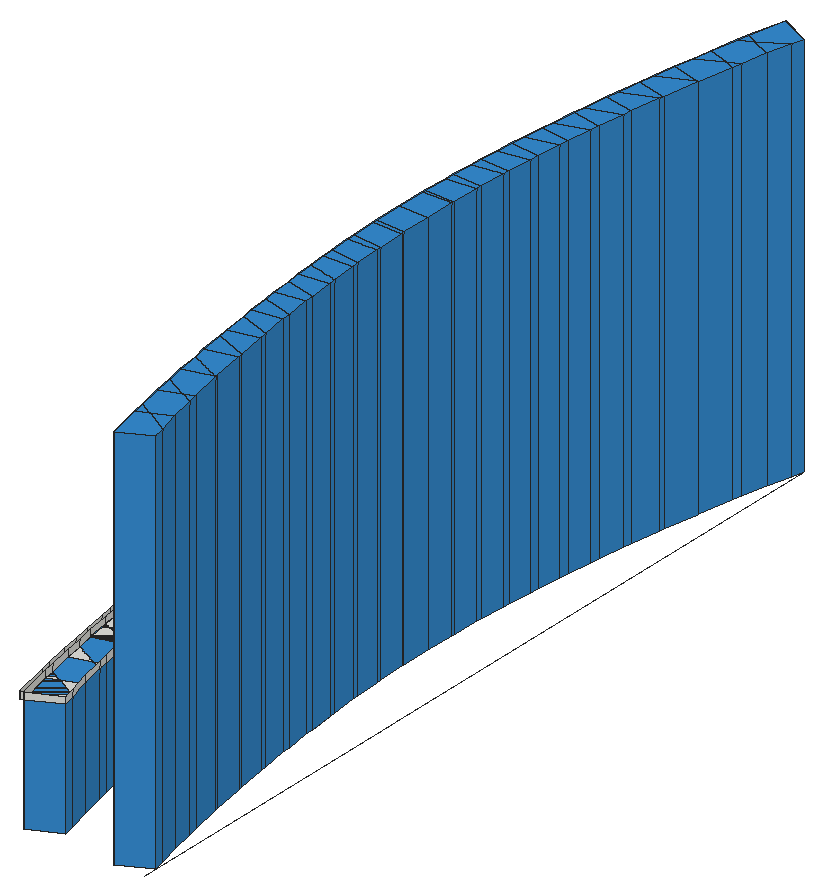
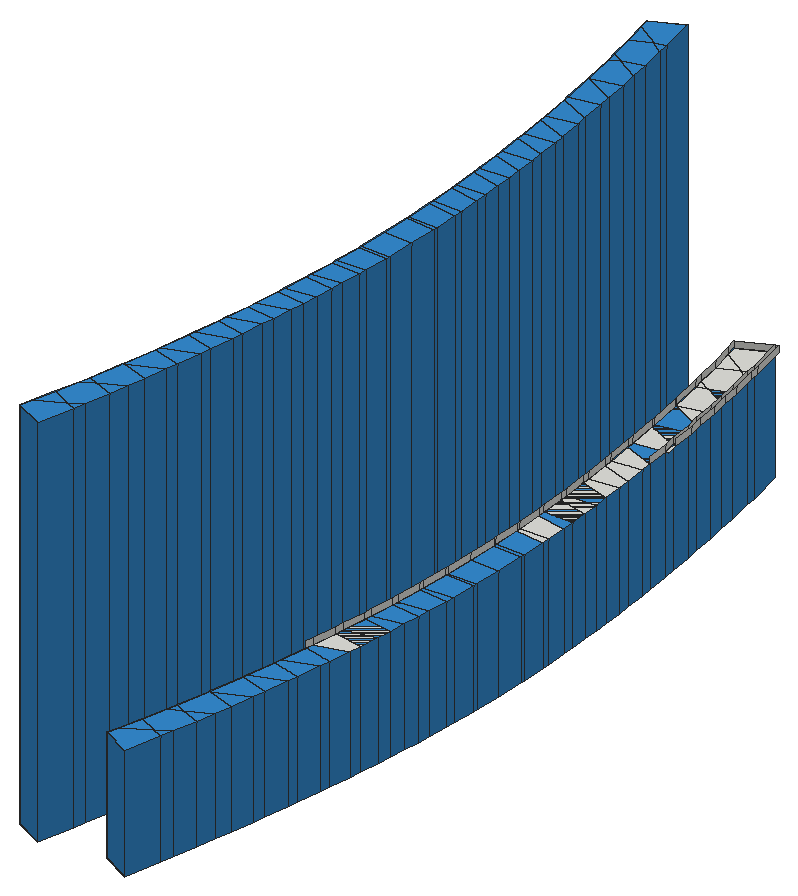
# SketchUp Ruby script. Lengths in inches.
U = 1.inch
M = Sketchup.active_model
def pt(a) = Geom::Point3d.new(a.map { |v| v * U })
def face(e, loops, mat)
  f = e.add_face(loops[0].map { |a| pt(a) })
  loops[1..].each { |l| e.add_face(l.map { |a| pt(a) }).erase! }
  f.material = f.back_material = mat if mat
  f
end
# faces: each face lists its corners as indices into pts; further lists are holes
def faces(e, pts, list, mat = nil) = list.each { |f| face(e, (f[0].is_a?(Array) ? f : [f]).map { |l| l.map { |i| pts[i] } }, mat) }
# xy, xz, yz: faces in a plane at the given z, y or x. An outline is a flat list of corners, or four numbers for a rectangle; further outlines are holes
def ring(l) = l.size == 4 ? [[l[0], l[1]], [l[2], l[1]], [l[2], l[3]], [l[0], l[3]]] : l.each_slice(2).to_a
def flat(e, list, mat, &to3) = list.each { |f| face(e, (f[0].is_a?(Array) ? f : [f]).map { |l| ring(l).map { |u, v| to3.(u, v) } }, mat) }
def xy(e, z, list, mat = nil) = flat(e, list, mat) { |x, y| [x, y, z] }
def xz(e, y, list, mat = nil) = flat(e, list, mat) { |x, z| [x, y, z] }
def yz(e, x, list, mat = nil) = flat(e, list, mat) { |y, z| [x, y, z] }
def lines(e, pts, list) = list.each { |a, b| e.add_line(pt(pts[a]), pt(pts[b])) }
# prism: a flat outline (further loops are holes) pulled along v
def prism(e, loops, v, mat = nil)
  f = face(e, loops, mat); d = Geom::Vector3d.new(v.map { |x| x * U })
  f.pushpull(f.normal.samedirection?(d) ? d.length : -d.length)
end
def box(e, o, s, mat = nil) = prism(e, [[o, [o[0] + s[0], o[1], o[2]], [o[0] + s[0], o[1] + s[1], o[2]], [o[0], o[1] + s[1], o[2]]]], [0, 0, s[2]], mat)
def at(x, y, z, deg = 0) = Geom::Transformation.translation(pt([x, y, z])) * Geom::Transformation.rotation(ORIGIN, Z_AXIS, deg.degrees)
def axes(o, x, y, z) = Geom::Transformation.new([*x, 0, *y, 0, *z, 0, *pt(o).to_a, 1])
def part(name) = M.definitions.add(name)
# library, detail: a bought-in or finely detailed component or shape, given as its bounding box
def library(name, o, s) = part(name).tap { |d| box(d.entities, o, s) }
def detail(e, o, s) = box(e.add_group.entities, o, s)
def put(e, d, t, mat = nil) = e.add_instance(d, t).tap { |i| i.material = mat if mat }
def group(e, t, mat = nil) = e.add_group.tap { |g| g.transformation = t; g.material = mat if mat }.entities
root = M.entities
M.materials.add("[Color I07]").color = [53, 140, 209]
xy(root,42,[[201.82,0,199.28,11.47,200.26,11.66,202.8,0.22],[202.8,0.22,200.26,11.66,203.64,12.99,211.37,8.47,212.15,4.84],[211.37,8.47,203.64,12.99,209.51,15.61],[199.28,11.47,198.66,15.15,199.65,15.33,200.26,11.66],[200.26,11.66,199.65,15.33,203.64,12.99],
  [203.64,12.99,199.65,15.33,198.01,23.07,204.28,25.25,207.95,23.33,209.51,15.61],[198.66,15.15,197.03,22.89,198.01,23.07,199.65,15.33],[197.03,22.89,196.1,28.84,197.09,29.01,198.01,23.07],[198.01,23.07,197.09,29.01,204.28,25.25],[207.95,23.33,204.28,25.25,207.19,26.4],
  [204.28,25.25,197.09,29.01,196,34.4,204.76,37.05,205.21,36.84,207.19,26.4],[196.1,28.84,195.01,34.23,196,34.4,197.09,29.01],[195.01,34.23,193.99,41.41,194.97,41.57,196,34.4],[196,34.4,194.97,41.57,204.76,37.05],[205.21,36.84,204.76,37.05,205.13,37.17],
  [204.76,37.05,194.97,41.57,194.2,45.63,203.24,47.92,205.13,37.17],[193.99,41.41,193.21,45.47,194.2,45.63,194.97,41.57],[193.21,45.47,192.21,53.1,193.2,53.25,194.2,45.63],[194.2,45.63,193.2,53.25,203.09,49.24,203.24,47.92],[203.09,49.24,193.2,53.25,192.58,56.72,201.57,58.57],
  [192.21,53.1,191.59,56.57,192.58,56.72,193.2,53.25],[192.58,56.72,191.71,64.21,201.35,60.83,201.57,58.57],[201.35,60.83,191.71,64.21,191.15,67.64,200.12,69.11],[191.15,67.64,190.46,74.59,199.89,71.79,200.12,69.11],[199.89,71.79,190.46,74.59,189.91,78.39,198.87,79.53],
  [189.91,78.39,189.43,84.51,198.7,82.24,198.87,79.53],[198.7,82.24,189.43,84.51,188.86,88.98,197.84,89.82],[188.86,88.98,188.59,94.0625,197.74,92.28,197.84,89.82],[197.74,92.28,188.59,94.0625,188.04,99.42,197.03,100.01],[188.04,99.42,187.93,103.33,197,102.01,197.03,100.01],
  [197,102.01,187.93,103.33,187.45,109.73,196.45,110.11],[187.45,109.73,187.45,112.39,196.46,111.52,196.45,110.11],[196.45,150.19,187.45,150.57,187.93,156.98,197,158.29],[187.93,156.98,188.04,160.89,197.03,160.29,197,158.29],[197.03,160.29,188.04,160.89,188.59,166.24,197.74,168.03],
  [188.59,166.24,188.86,171.33,197.84,170.48,197.74,168.03],[197.84,170.48,188.86,171.33,189.43,175.79,198.7,178.07],[189.43,175.79,189.91,181.91,198.87,180.78,198.7,178.07],[198.87,180.78,189.91,181.91,190.46,185.71,199.89,188.52],[190.46,185.71,191.15,192.67,200.12,191.2,199.89,188.52]])
p = [[201.82,0,44],[199.28,11.47,44],[199.28,11.47,42],[201.82,0,42],[202.8,0.22,44],[202.8,0.22,42],
  [200.26,11.66,42],[200.26,11.66,44],[212.15,4.84,42],[212.15,4.84,44],[211.37,8.47,42],[211.37,8.47,44],
  [209.51,15.61,42],[209.51,15.61,44],[198.66,15.15,44],[198.66,15.15,42],[199.65,15.33,42],[199.65,15.33,44],
  [197.03,22.89,44],[197.03,22.89,42],[198.01,23.07,42],[198.01,23.07,44],[207.95,23.33,42],[207.95,23.33,44],
  [196.1,28.84,44],[196.1,28.84,42],[197.09,29.01,42],[197.09,29.01,44],[207.19,26.4,42],[207.19,26.4,44],
  [205.21,36.84,42],[205.21,36.84,44],[195.01,34.23,44],[195.01,34.23,42],[196,34.4,42],[196,34.4,44],
  [193.99,41.41,44],[193.99,41.41,42],[194.97,41.57,42],[194.97,41.57,44],[205.13,37.17,42],[205.13,37.17,44],
  [203.24,47.92,42],[203.24,47.92,44],[193.21,45.47,44],[193.21,45.47,42],[194.2,45.63,42],[194.2,45.63,44],
  [192.21,53.1,44],[192.21,53.1,42],[193.2,53.25,42],[193.2,53.25,44],[203.09,49.24,42],[203.09,49.24,44],
  [201.57,58.57,42],[201.57,58.57,44],[192.58,56.72,42],[192.58,56.72,44],[191.71,64.21,42],[191.71,64.21,44],
  [201.35,60.83,42],[201.35,60.83,44],[200.12,69.11,42],[200.12,69.11,44],[199.89,71.79,42],[199.89,71.79,44],
  [198.87,79.53,42],[198.87,79.53,44],[198.7,82.24,42],[198.7,82.24,44],[197.84,89.82,42],[197.84,89.82,44],
  [197.74,92.28,42],[197.74,92.28,44],[197.03,100.01,42],[197.03,100.01,44],[197,102.01,42],[197,102.01,44],
  [196.45,110.11,42],[196.45,110.11,44],[196.46,111.52,42],[196.46,111.52,44],[196.11,120.15,42],[196.11,120.15,44],
  [196.13,120.87,42],[196.13,120.87,44],[196.01,130.15,42],[196.01,130.15,44],[196.13,139.43,42],[196.13,139.43,44],
  [196.11,140.16,42],[196.11,140.16,44],[196.46,148.79,42],[196.46,148.79,44],[196.45,150.19,42],[196.45,150.19,44],
  [197,158.29,42],[197,158.29,44],[197.03,160.29,42],[197.03,160.29,44],[197.74,168.03,42],[197.74,168.03,44],
  [197.84,170.48,42],[197.84,170.48,44],[198.7,178.07,42],[198.7,178.07,44],[198.87,180.78,42],[198.87,180.78,44],
  [199.89,188.52,42],[199.89,188.52,44],[200.12,191.2,42],[200.12,191.2,44],[240,255.46,6],[240,0.22,6]]
faces(root,p,[[0,1,2,3],[4,0,3,5],[4,5,6,7],[8,9,4,5],[10,11,9,8],[12,13,11,10],[1,14,15,2],[7,6,16,17],
  [14,18,19,15],[17,16,20,21],[22,23,13,12],[18,24,25,19],[21,20,26,27],[28,29,23,22],[30,31,29,28],[24,32,33,25],
  [27,26,34,35],[32,36,37,33],[35,34,38,39],[40,41,31,30],[42,43,41,40],[36,44,45,37],[39,38,46,47],[44,48,49,45],
  [47,46,50,51],[52,53,43,42],[54,55,53,52],[51,50,56,57],[57,56,58,59],[60,61,55,54],[62,63,61,60],[64,65,63,62],
  [66,67,65,64],[68,69,67,66],[70,71,69,68],[72,73,71,70],[74,75,73,72],[76,77,75,74],[78,79,77,76],[80,81,79,78],
  [82,83,81,80],[84,85,83,82],[86,87,85,84],[88,89,87,86],[90,91,89,88],[92,93,91,90],[94,95,93,92],[96,97,95,94],
  [98,99,97,96],[100,101,99,98],[102,103,101,100],[104,105,103,102],[106,107,105,104],[108,109,107,106],[110,111,109,108]])
lines(root,p,[[112,113]])
g1 = group(root,at(196.01,10.15,6,90),"[Color I07]")
xy(g1,0,[[-5.31,-16.14,-9.9375,-6.79,1.5,-4.25,2.84,-7.63,-1.69,-15.36],[245.31,-16.14,241.69,-15.36,237.16,-7.63,238.5,-4.25,249.9375,-6.79],[-1.69,-15.36,2.84,-7.63,5.46,-13.51],[241.69,-15.36,234.54,-13.51,237.16,-7.63],[5.46,-13.51,2.84,-7.63,5.18,-3.64,12.91,-2,15.1,-8.28,13.18,-11.94],
  [234.54,-13.51,226.82,-11.94,224.9,-8.28,227.09,-2,234.82,-3.64,237.16,-7.63],[13.18,-11.94,15.1,-8.28,16.25,-11.18],[226.82,-11.94,223.75,-11.18,224.9,-8.28],[16.25,-11.18,15.1,-8.28,18.86,-1.08,24.25,0.01,26.89,-8.75,26.68,-9.2],[223.75,-11.18,213.32,-9.2,213.11,-8.75,215.75,0.01,221.14,-1.08,224.9,-8.28],
  [26.68,-9.2,26.89,-8.75,27.02,-9.125],[213.32,-9.2,212.98,-9.125,213.11,-8.75],[27.02,-9.125,26.89,-8.75,31.42,1.03,35.48,1.8125,37.76,-7.24],[212.98,-9.125,202.24,-7.24,204.52,1.8125,208.58,1.03,213.11,-8.75],[26.89,-8.75,24.25,0.01,31.42,1.03],
  [213.11,-8.75,208.58,1.03,215.75,0.01],[15.1,-8.28,12.91,-2,18.86,-1.08],[224.9,-8.28,221.14,-1.08,227.09,-2],[2.84,-7.63,1.5,-4.25,5.18,-3.64],[237.16,-7.63,234.82,-3.64,238.5,-4.25],
  [37.76,-7.24,35.48,1.8125,43.1,2.81,39.08,-7.09],[202.24,-7.24,200.92,-7.09,196.9,2.81,204.52,1.8125],[39.08,-7.09,43.1,2.81,46.5625,3.43,48.42,-5.57],[200.92,-7.09,191.58,-5.57,193.4375,3.43,196.9,2.81],[48.42,-5.57,46.5625,3.43,54.06,4.29,50.68,-5.34],
  [191.58,-5.57,189.32,-5.34,185.94,4.29,193.4375,3.43],[50.68,-5.34,54.06,4.29,57.49,4.86,58.95,-4.11],[189.32,-5.34,181.05,-4.11,182.51,4.86,185.94,4.29],[58.95,-4.11,57.49,4.86,64.44,5.54,61.64,-3.89],[181.05,-4.11,178.36,-3.89,175.56,5.54,182.51,4.86],
  [61.64,-3.89,64.44,5.54,68.24,6.1,69.37,-2.87],[178.36,-3.89,170.63,-2.87,171.76,6.1,175.56,5.54],[69.37,-2.87,68.24,6.1,74.36,6.58,72.08,-2.69],[170.63,-2.87,167.92,-2.69,165.64,6.58,171.76,6.1],[72.08,-2.69,74.36,6.58,78.83,7.14,79.67,-1.84],
  [167.92,-2.69,160.33,-1.84,161.17,7.14,165.64,6.58],[79.67,-1.84,78.83,7.14,83.91,7.42,82.125,-1.73],[160.33,-1.84,157.875,-1.73,156.09,7.42,161.17,7.14],[82.125,-1.73,83.91,7.42,89.26,7.97,89.86,-1.03],[157.875,-1.73,150.14,-1.03,150.74,7.97,156.09,7.42],
  [89.86,-1.03,89.26,7.97,93.18,8.07,91.86,-0.99],[150.14,-1.03,148.14,-0.99,146.82,8.07,150.74,7.97],[91.86,-0.99,93.18,8.07,99.58,8.56,99.96,-0.45],[148.14,-0.99,140.04,-0.45,140.42,8.56,146.82,8.07],[101.36,-0.46,99.96,-0.45,99.58,8.56,102.23,8.55],
  [101.36,-0.46,102.23,8.55,109.8125,8.91,110,-0.1],[138.64,-0.46,130,-0.1,130.1875,8.91,137.77,8.55],[138.64,-0.46,137.77,8.55,140.42,8.56,140.04,-0.45],[110.72,-0.13,110,-0.1,109.8125,8.91,111.15,8.86],[110.72,-0.13,111.15,8.86,120,9,120,0],
  [129.28,-0.13,120,0,120,9,128.85,8.86],[129.28,-0.13,128.85,8.86,130.1875,8.91,130,-0.1]])
xy(g1,36,[[-5.31,-16.14,-1.69,-15.36,2.84,-7.63,1.5,-4.25,-9.9375,-6.79],[245.31,-16.14,249.9375,-6.79,238.5,-4.25,237.16,-7.63,241.69,-15.36],[-1.69,-15.36,5.46,-13.51,2.84,-7.63],[241.69,-15.36,237.16,-7.63,234.54,-13.51],[5.46,-13.51,13.18,-11.94,15.1,-8.28,12.91,-2,5.18,-3.64,2.84,-7.63],
  [234.54,-13.51,237.16,-7.63,234.82,-3.64,227.09,-2,224.9,-8.28,226.82,-11.94],[13.18,-11.94,16.25,-11.18,15.1,-8.28],[226.82,-11.94,224.9,-8.28,223.75,-11.18],[16.25,-11.18,26.68,-9.2,26.89,-8.75,24.25,0.01,18.86,-1.08,15.1,-8.28],[223.75,-11.18,224.9,-8.28,221.14,-1.08,215.75,0.01,213.11,-8.75,213.32,-9.2],
  [26.68,-9.2,27.02,-9.125,26.89,-8.75],[213.32,-9.2,213.11,-8.75,212.98,-9.125],[27.02,-9.125,37.76,-7.24,35.48,1.8125,31.42,1.03,26.89,-8.75],[212.98,-9.125,213.11,-8.75,208.58,1.03,204.52,1.8125,202.24,-7.24],[26.89,-8.75,31.42,1.03,24.25,0.01],
  [213.11,-8.75,215.75,0.01,208.58,1.03],[15.1,-8.28,18.86,-1.08,12.91,-2],[224.9,-8.28,227.09,-2,221.14,-1.08],[2.84,-7.63,5.18,-3.64,1.5,-4.25],[237.16,-7.63,238.5,-4.25,234.82,-3.64],
  [37.76,-7.24,39.08,-7.09,43.1,2.81,35.48,1.8125],[202.24,-7.24,204.52,1.8125,196.9,2.81,200.92,-7.09],[39.08,-7.09,48.42,-5.57,46.5625,3.43,43.1,2.81],[200.92,-7.09,196.9,2.81,193.4375,3.43,191.58,-5.57],[48.42,-5.57,50.68,-5.34,54.06,4.29,46.5625,3.43],
  [191.58,-5.57,193.4375,3.43,185.94,4.29,189.32,-5.34],[50.68,-5.34,58.95,-4.11,57.49,4.86,54.06,4.29],[189.32,-5.34,185.94,4.29,182.51,4.86,181.05,-4.11],[58.95,-4.11,61.64,-3.89,64.44,5.54,57.49,4.86],[181.05,-4.11,182.51,4.86,175.56,5.54,178.36,-3.89],
  [61.64,-3.89,69.37,-2.87,68.24,6.1,64.44,5.54],[178.36,-3.89,175.56,5.54,171.76,6.1,170.63,-2.87],[69.37,-2.87,72.08,-2.69,74.36,6.58,68.24,6.1],[170.63,-2.87,171.76,6.1,165.64,6.58,167.92,-2.69],[72.08,-2.69,79.67,-1.84,78.83,7.14,74.36,6.58],
  [167.92,-2.69,165.64,6.58,161.17,7.14,160.33,-1.84],[79.67,-1.84,82.125,-1.73,83.91,7.42,78.83,7.14],[160.33,-1.84,161.17,7.14,156.09,7.42,157.875,-1.73],[82.125,-1.73,89.86,-1.03,89.26,7.97,83.91,7.42],[157.875,-1.73,156.09,7.42,150.74,7.97,150.14,-1.03],
  [89.86,-1.03,91.86,-0.99,93.18,8.07,89.26,7.97],[150.14,-1.03,150.74,7.97,146.82,8.07,148.14,-0.99],[91.86,-0.99,99.96,-0.45,99.58,8.56,93.18,8.07],[148.14,-0.99,146.82,8.07,140.42,8.56,140.04,-0.45],[101.36,-0.46,102.23,8.55,99.58,8.56,99.96,-0.45],
  [101.36,-0.46,110,-0.1,109.8125,8.91,102.23,8.55],[138.64,-0.46,137.77,8.55,130.1875,8.91,130,-0.1],[138.64,-0.46,140.04,-0.45,140.42,8.56,137.77,8.55],[110.72,-0.13,111.15,8.86,109.8125,8.91,110,-0.1],[110.72,-0.13,120,0,120,9,111.15,8.86],
  [129.28,-0.13,128.85,8.86,120,9,120,0],[129.28,-0.13,130,-0.1,130.1875,8.91,128.85,8.86]])
p = [[-5.31,-16.14,0],[-5.31,-16.14,36],[-9.9375,-6.79,36],[-9.9375,-6.79,0],[-1.69,-15.36,0],[-1.69,-15.36,36],
  [245.31,-16.14,0],[245.31,-16.14,36],[241.69,-15.36,36],[241.69,-15.36,0],[249.9375,-6.79,0],[249.9375,-6.79,36],
  [5.46,-13.51,0],[5.46,-13.51,36],[234.54,-13.51,36],[234.54,-13.51,0],[13.18,-11.94,0],[13.18,-11.94,36],
  [226.82,-11.94,36],[226.82,-11.94,0],[16.25,-11.18,0],[16.25,-11.18,36],[223.75,-11.18,36],[223.75,-11.18,0],
  [26.68,-9.2,0],[26.68,-9.2,36],[213.32,-9.2,36],[213.32,-9.2,0],[27.02,-9.125,0],[27.02,-9.125,36],
  [212.98,-9.125,36],[212.98,-9.125,0],[37.76,-7.24,0],[37.76,-7.24,36],[202.24,-7.24,36],[202.24,-7.24,0],
  [39.08,-7.09,0],[39.08,-7.09,36],[200.92,-7.09,36],[200.92,-7.09,0],[48.42,-5.57,0],[48.42,-5.57,36],
  [191.58,-5.57,36],[191.58,-5.57,0],[1.5,-4.25,36],[1.5,-4.25,0],[238.5,-4.25,0],[238.5,-4.25,36],
  [50.68,-5.34,0],[50.68,-5.34,36],[189.32,-5.34,36],[189.32,-5.34,0],[58.95,-4.11,0],[58.95,-4.11,36],
  [181.05,-4.11,36],[181.05,-4.11,0],[5.18,-3.64,36],[5.18,-3.64,0],[234.82,-3.64,0],[234.82,-3.64,36],
  [61.64,-3.89,0],[61.64,-3.89,36],[178.36,-3.89,36],[178.36,-3.89,0],[69.37,-2.87,0],[69.37,-2.87,36],
  [170.63,-2.87,36],[170.63,-2.87,0],[12.91,-2,36],[12.91,-2,0],[227.09,-2,0],[227.09,-2,36],
  [72.08,-2.69,0],[72.08,-2.69,36],[167.92,-2.69,36],[167.92,-2.69,0],[79.67,-1.84,0],[79.67,-1.84,36],
  [160.33,-1.84,36],[160.33,-1.84,0],[18.86,-1.08,36],[18.86,-1.08,0],[221.14,-1.08,0],[221.14,-1.08,36],
  [82.125,-1.73,0],[82.125,-1.73,36],[157.875,-1.73,36],[157.875,-1.73,0],[89.86,-1.03,0],[89.86,-1.03,36],
  [150.14,-1.03,36],[150.14,-1.03,0],[24.25,0.01,36],[24.25,0.01,0],[215.75,0.01,0],[215.75,0.01,36],
  [91.86,-0.99,0],[91.86,-0.99,36],[99.96,-0.45,0],[99.96,-0.45,36],[148.14,-0.99,0],[148.14,-0.99,36],
  [140.04,-0.45,36],[140.04,-0.45,0],[101.36,-0.46,0],[101.36,-0.46,36],[110,-0.1,0],[110,-0.1,36],
  [138.64,-0.46,0],[138.64,-0.46,36],[130,-0.1,36],[130,-0.1,0],[110.72,-0.13,0],[110.72,-0.13,36],
  [120,0,0],[120,0,36],[129.28,-0.13,0],[129.28,-0.13,36],[31.42,1.03,36],[31.42,1.03,0],
  [208.58,1.03,0],[208.58,1.03,36],[35.48,1.8125,36],[35.48,1.8125,0],[204.52,1.8125,0],[204.52,1.8125,36],
  [43.1,2.81,36],[43.1,2.81,0],[196.9,2.81,0],[196.9,2.81,36],[46.5625,3.43,36],[46.5625,3.43,0],
  [193.4375,3.43,0],[193.4375,3.43,36],[54.06,4.29,36],[54.06,4.29,0],[185.94,4.29,0],[185.94,4.29,36],
  [57.49,4.86,36],[57.49,4.86,0],[182.51,4.86,0],[182.51,4.86,36],[64.44,5.54,36],[64.44,5.54,0],
  [175.56,5.54,0],[175.56,5.54,36],[68.24,6.1,36],[68.24,6.1,0],[171.76,6.1,0],[171.76,6.1,36],
  [74.36,6.58,36],[74.36,6.58,0],[165.64,6.58,0],[165.64,6.58,36],[78.83,7.14,36],[78.83,7.14,0],
  [161.17,7.14,0],[161.17,7.14,36],[83.91,7.42,36],[83.91,7.42,0],[156.09,7.42,0],[156.09,7.42,36],
  [89.26,7.97,36],[89.26,7.97,0],[150.74,7.97,0],[150.74,7.97,36],[93.18,8.07,36],[93.18,8.07,0],
  [146.82,8.07,0],[146.82,8.07,36],[99.58,8.56,36],[99.58,8.56,0],[140.42,8.56,0],[140.42,8.56,36],
  [102.23,8.55,36],[102.23,8.55,0],[109.8125,8.91,36],[109.8125,8.91,0],[130.1875,8.91,0],[130.1875,8.91,36],
  [137.77,8.55,36],[137.77,8.55,0],[111.15,8.86,36],[111.15,8.86,0],[120,9,36],[120,9,0],
  [128.85,8.86,36],[128.85,8.86,0]]
faces(g1,p,[[0,1,2,3],[0,4,5,1],[6,7,8,9],[10,11,7,6],[4,12,13,5],[9,8,14,15],[12,16,17,13],[15,14,18,19],
  [16,20,21,17],[19,18,22,23],[24,25,21,20],[23,22,26,27],[28,29,25,24],[27,26,30,31],[32,33,29,28],[31,30,34,35],
  [36,37,33,32],[35,34,38,39],[40,41,37,36],[39,38,42,43],[3,2,44,45],[10,46,47,11],[48,49,41,40],[43,42,50,51],
  [52,53,49,48],[51,50,54,55],[45,44,56,57],[46,58,59,47],[60,61,53,52],[55,54,62,63],[64,65,61,60],[63,62,66,67],
  [57,56,68,69],[58,70,71,59],[72,73,65,64],[67,66,74,75],[76,77,73,72],[75,74,78,79],[69,68,80,81],[82,83,71,70],
  [84,85,77,76],[79,78,86,87],[88,89,85,84],[87,86,90,91],[81,80,92,93],[94,95,83,82],[96,97,89,88],[98,99,97,96],
  [100,101,102,103],[91,90,101,100],[104,105,99,98],[106,107,105,104],[108,109,110,111],[103,102,109,108],[112,113,107,106],[114,115,113,112],
  [116,117,115,114],[111,110,117,116],[93,92,118,119],[120,121,95,94],[119,118,122,123],[124,125,121,120],[123,122,126,127],[128,129,125,124],
  [127,126,130,131],[132,133,129,128],[131,130,134,135],[136,137,133,132],[135,134,138,139],[140,141,137,136],[139,138,142,143],[144,145,141,140],
  [143,142,146,147],[148,149,145,144],[147,146,150,151],[152,153,149,148],[151,150,154,155],[152,156,157,153],[155,154,158,159],[160,161,157,156],
  [159,158,162,163],[164,165,161,160],[163,162,166,167],[168,169,165,164],[167,166,170,171],[172,173,169,168],[171,170,174,175],[175,174,176,177],
  [178,179,180,181],[181,180,173,172],[177,176,182,183],[183,182,184,185],[185,184,186,187],[187,186,179,178]])
g2 = group(root,at(223.86,10.15,6,90),"[Color I07]")
xy(g2,0,[[-5.31,-16.14,-9.9375,-6.79,1.5,-4.25,2.84,-7.63,-1.69,-15.36],[245.31,-16.14,241.69,-15.36,237.16,-7.63,238.5,-4.25,249.9375,-6.79],[-1.69,-15.36,2.84,-7.63,5.46,-13.51],[241.69,-15.36,234.54,-13.51,237.16,-7.63],[5.46,-13.51,2.84,-7.63,5.18,-3.64,12.91,-2,15.1,-8.28,13.18,-11.94],
  [234.54,-13.51,226.82,-11.94,224.9,-8.28,227.09,-2,234.82,-3.64,237.16,-7.63],[13.18,-11.94,15.1,-8.28,16.25,-11.18],[226.82,-11.94,223.75,-11.18,224.9,-8.28],[16.25,-11.18,15.1,-8.28,18.86,-1.08,24.25,0.01,26.89,-8.75,26.68,-9.2],[223.75,-11.18,213.32,-9.2,213.11,-8.75,215.75,0.01,221.14,-1.08,224.9,-8.28],
  [26.68,-9.2,26.89,-8.75,27.02,-9.125],[213.32,-9.2,212.98,-9.125,213.11,-8.75],[27.02,-9.125,26.89,-8.75,31.42,1.03,35.48,1.8125,37.76,-7.24],[212.98,-9.125,202.24,-7.24,204.52,1.8125,208.58,1.03,213.11,-8.75],[26.89,-8.75,24.25,0.01,31.42,1.03],
  [213.11,-8.75,208.58,1.03,215.75,0.01],[15.1,-8.28,12.91,-2,18.86,-1.08],[224.9,-8.28,221.14,-1.08,227.09,-2],[2.84,-7.63,1.5,-4.25,5.18,-3.64],[237.16,-7.63,234.82,-3.64,238.5,-4.25],
  [37.76,-7.24,35.48,1.8125,43.1,2.81,39.08,-7.09],[202.24,-7.24,200.92,-7.09,196.9,2.81,204.52,1.8125],[39.08,-7.09,43.1,2.81,46.5625,3.43,48.42,-5.57],[200.92,-7.09,191.58,-5.57,193.4375,3.43,196.9,2.81],[48.42,-5.57,46.5625,3.43,54.06,4.29,50.68,-5.34],
  [191.58,-5.57,189.32,-5.34,185.94,4.29,193.4375,3.43],[50.68,-5.34,54.06,4.29,57.49,4.86,58.95,-4.11],[189.32,-5.34,181.05,-4.11,182.51,4.86,185.94,4.29],[58.95,-4.11,57.49,4.86,64.44,5.54,61.64,-3.89],[181.05,-4.11,178.36,-3.89,175.56,5.54,182.51,4.86],
  [61.64,-3.89,64.44,5.54,68.24,6.1,69.37,-2.87],[178.36,-3.89,170.63,-2.87,171.76,6.1,175.56,5.54],[69.37,-2.87,68.24,6.1,74.36,6.58,72.08,-2.69],[170.63,-2.87,167.92,-2.69,165.64,6.58,171.76,6.1],[72.08,-2.69,74.36,6.58,78.83,7.14,79.67,-1.84],
  [167.92,-2.69,160.33,-1.84,161.17,7.14,165.64,6.58],[79.67,-1.84,78.83,7.14,83.91,7.42,82.125,-1.73],[160.33,-1.84,157.875,-1.73,156.09,7.42,161.17,7.14],[82.125,-1.73,83.91,7.42,89.26,7.97,89.86,-1.03],[157.875,-1.73,150.14,-1.03,150.74,7.97,156.09,7.42],
  [89.86,-1.03,89.26,7.97,93.18,8.07,91.86,-0.99],[150.14,-1.03,148.14,-0.99,146.82,8.07,150.74,7.97],[91.86,-0.99,93.18,8.07,99.58,8.56,99.96,-0.45],[148.14,-0.99,140.04,-0.45,140.42,8.56,146.82,8.07],[101.36,-0.46,99.96,-0.45,99.58,8.56,102.23,8.55],
  [101.36,-0.46,102.23,8.55,109.8125,8.91,110,-0.1],[138.64,-0.46,130,-0.1,130.1875,8.91,137.77,8.55],[138.64,-0.46,137.77,8.55,140.42,8.56,140.04,-0.45],[110.72,-0.13,110,-0.1,109.8125,8.91,111.15,8.86],[110.72,-0.13,111.15,8.86,120,9,120,0],
  [129.28,-0.13,120,0,120,9,128.85,8.86],[129.28,-0.13,128.85,8.86,130.1875,8.91,130,-0.1]])
xy(g2,120,[[-5.31,-16.14,-1.69,-15.36,2.84,-7.63,1.5,-4.25,-9.9375,-6.79],[245.31,-16.14,249.9375,-6.79,238.5,-4.25,237.16,-7.63,241.69,-15.36],[-1.69,-15.36,5.46,-13.51,2.84,-7.63],[241.69,-15.36,237.16,-7.63,234.54,-13.51],[5.46,-13.51,13.18,-11.94,15.1,-8.28,12.91,-2,5.18,-3.64,2.84,-7.63],
  [234.54,-13.51,237.16,-7.63,234.82,-3.64,227.09,-2,224.9,-8.28,226.82,-11.94],[13.18,-11.94,16.25,-11.18,15.1,-8.28],[226.82,-11.94,224.9,-8.28,223.75,-11.18],[16.25,-11.18,26.68,-9.2,26.89,-8.75,24.25,0.01,18.86,-1.08,15.1,-8.28],[223.75,-11.18,224.9,-8.28,221.14,-1.08,215.75,0.01,213.11,-8.75,213.32,-9.2],
  [26.68,-9.2,27.02,-9.125,26.89,-8.75],[213.32,-9.2,213.11,-8.75,212.98,-9.125],[27.02,-9.125,37.76,-7.24,35.48,1.8125,31.42,1.03,26.89,-8.75],[212.98,-9.125,213.11,-8.75,208.58,1.03,204.52,1.8125,202.24,-7.24],[26.89,-8.75,31.42,1.03,24.25,0.01],
  [213.11,-8.75,215.75,0.01,208.58,1.03],[15.1,-8.28,18.86,-1.08,12.91,-2],[224.9,-8.28,227.09,-2,221.14,-1.08],[2.84,-7.63,5.18,-3.64,1.5,-4.25],[237.16,-7.63,238.5,-4.25,234.82,-3.64],
  [37.76,-7.24,39.08,-7.09,43.1,2.81,35.48,1.8125],[202.24,-7.24,204.52,1.8125,196.9,2.81,200.92,-7.09],[39.08,-7.09,48.42,-5.57,46.5625,3.43,43.1,2.81],[200.92,-7.09,196.9,2.81,193.4375,3.43,191.58,-5.57],[48.42,-5.57,50.68,-5.34,54.06,4.29,46.5625,3.43],
  [191.58,-5.57,193.4375,3.43,185.94,4.29,189.32,-5.34],[50.68,-5.34,58.95,-4.11,57.49,4.86,54.06,4.29],[189.32,-5.34,185.94,4.29,182.51,4.86,181.05,-4.11],[58.95,-4.11,61.64,-3.89,64.44,5.54,57.49,4.86],[181.05,-4.11,182.51,4.86,175.56,5.54,178.36,-3.89],
  [61.64,-3.89,69.37,-2.87,68.24,6.1,64.44,5.54],[178.36,-3.89,175.56,5.54,171.76,6.1,170.63,-2.87],[69.37,-2.87,72.08,-2.69,74.36,6.58,68.24,6.1],[170.63,-2.87,171.76,6.1,165.64,6.58,167.92,-2.69],[72.08,-2.69,79.67,-1.84,78.83,7.14,74.36,6.58],
  [167.92,-2.69,165.64,6.58,161.17,7.14,160.33,-1.84],[79.67,-1.84,82.125,-1.73,83.91,7.42,78.83,7.14],[160.33,-1.84,161.17,7.14,156.09,7.42,157.875,-1.73],[82.125,-1.73,89.86,-1.03,89.26,7.97,83.91,7.42],[157.875,-1.73,156.09,7.42,150.74,7.97,150.14,-1.03],
  [89.86,-1.03,91.86,-0.99,93.18,8.07,89.26,7.97],[150.14,-1.03,150.74,7.97,146.82,8.07,148.14,-0.99],[91.86,-0.99,99.96,-0.45,99.58,8.56,93.18,8.07],[148.14,-0.99,146.82,8.07,140.42,8.56,140.04,-0.45],[101.36,-0.46,102.23,8.55,99.58,8.56,99.96,-0.45],
  [101.36,-0.46,110,-0.1,109.8125,8.91,102.23,8.55],[138.64,-0.46,137.77,8.55,130.1875,8.91,130,-0.1],[138.64,-0.46,140.04,-0.45,140.42,8.56,137.77,8.55],[110.72,-0.13,111.15,8.86,109.8125,8.91,110,-0.1],[110.72,-0.13,120,0,120,9,111.15,8.86],
  [129.28,-0.13,128.85,8.86,120,9,120,0],[129.28,-0.13,130,-0.1,130.1875,8.91,128.85,8.86]])
p = [[-5.31,-16.14,0],[-5.31,-16.14,120],[-9.9375,-6.79,120],[-9.9375,-6.79,0],[-1.69,-15.36,0],[-1.69,-15.36,120],
  [245.31,-16.14,120],[241.69,-15.36,120],[241.69,-15.36,0],[245.31,-16.14,0],[249.9375,-6.79,0],[249.9375,-6.79,120],
  [5.46,-13.51,0],[5.46,-13.51,120],[234.54,-13.51,120],[234.54,-13.51,0],[13.18,-11.94,0],[13.18,-11.94,120],
  [226.82,-11.94,120],[226.82,-11.94,0],[16.25,-11.18,0],[16.25,-11.18,120],[223.75,-11.18,120],[223.75,-11.18,0],
  [26.68,-9.2,0],[26.68,-9.2,120],[213.32,-9.2,120],[213.32,-9.2,0],[27.02,-9.125,0],[27.02,-9.125,120],
  [212.98,-9.125,120],[212.98,-9.125,0],[37.76,-7.24,0],[37.76,-7.24,120],[202.24,-7.24,120],[202.24,-7.24,0],
  [39.08,-7.09,0],[39.08,-7.09,120],[200.92,-7.09,120],[200.92,-7.09,0],[48.42,-5.57,0],[48.42,-5.57,120],
  [191.58,-5.57,120],[191.58,-5.57,0],[1.5,-4.25,120],[1.5,-4.25,0],[238.5,-4.25,0],[238.5,-4.25,120],
  [50.68,-5.34,0],[50.68,-5.34,120],[189.32,-5.34,120],[189.32,-5.34,0],[58.95,-4.11,0],[58.95,-4.11,120],
  [181.05,-4.11,120],[181.05,-4.11,0],[5.18,-3.64,120],[5.18,-3.64,0],[234.82,-3.64,0],[234.82,-3.64,120],
  [61.64,-3.89,0],[61.64,-3.89,120],[178.36,-3.89,120],[178.36,-3.89,0],[69.37,-2.87,0],[69.37,-2.87,120],
  [170.63,-2.87,120],[170.63,-2.87,0],[12.91,-2,120],[12.91,-2,0],[227.09,-2,0],[227.09,-2,120],
  [72.08,-2.69,0],[72.08,-2.69,120],[167.92,-2.69,120],[167.92,-2.69,0],[79.67,-1.84,0],[79.67,-1.84,120],
  [160.33,-1.84,120],[160.33,-1.84,0],[18.86,-1.08,120],[18.86,-1.08,0],[221.14,-1.08,0],[221.14,-1.08,120],
  [82.125,-1.73,0],[82.125,-1.73,120],[157.875,-1.73,120],[157.875,-1.73,0],[89.86,-1.03,0],[89.86,-1.03,120],
  [150.14,-1.03,120],[150.14,-1.03,0],[24.25,0.01,120],[24.25,0.01,0],[215.75,0.01,0],[215.75,0.01,120],
  [91.86,-0.99,0],[91.86,-0.99,120],[99.96,-0.45,0],[99.96,-0.45,120],[148.14,-0.99,0],[148.14,-0.99,120],
  [140.04,-0.45,120],[140.04,-0.45,0],[101.36,-0.46,0],[101.36,-0.46,120],[110,-0.1,0],[110,-0.1,120],
  [138.64,-0.46,0],[138.64,-0.46,120],[130,-0.1,120],[130,-0.1,0],[110.72,-0.13,0],[110.72,-0.13,120],
  [120,0,0],[120,0,120],[129.28,-0.13,0],[129.28,-0.13,120],[31.42,1.03,120],[31.42,1.03,0],
  [208.58,1.03,0],[208.58,1.03,120],[35.48,1.8125,120],[35.48,1.8125,0],[204.52,1.8125,0],[204.52,1.8125,120],
  [43.1,2.81,120],[43.1,2.81,0],[196.9,2.81,0],[196.9,2.81,120],[46.5625,3.43,120],[46.5625,3.43,0],
  [193.4375,3.43,0],[193.4375,3.43,120],[54.06,4.29,120],[54.06,4.29,0],[185.94,4.29,0],[185.94,4.29,120],
  [57.49,4.86,120],[57.49,4.86,0],[182.51,4.86,0],[182.51,4.86,120],[64.44,5.54,120],[64.44,5.54,0],
  [175.56,5.54,0],[175.56,5.54,120],[68.24,6.1,120],[68.24,6.1,0],[171.76,6.1,0],[171.76,6.1,120],
  [74.36,6.58,120],[74.36,6.58,0],[165.64,6.58,0],[165.64,6.58,120],[78.83,7.14,120],[78.83,7.14,0],
  [161.17,7.14,0],[161.17,7.14,120],[83.91,7.42,120],[83.91,7.42,0],[156.09,7.42,0],[156.09,7.42,120],
  [89.26,7.97,120],[89.26,7.97,0],[150.74,7.97,0],[150.74,7.97,120],[93.18,8.07,120],[93.18,8.07,0],
  [146.82,8.07,0],[146.82,8.07,120],[99.58,8.56,120],[99.58,8.56,0],[140.42,8.56,0],[140.42,8.56,120],
  [102.23,8.55,120],[102.23,8.55,0],[109.8125,8.91,120],[109.8125,8.91,0],[130.1875,8.91,0],[130.1875,8.91,120],
  [137.77,8.55,120],[137.77,8.55,0],[111.15,8.86,120],[111.15,8.86,0],[120,9,120],[120,9,0],
  [128.85,8.86,120],[128.85,8.86,0]]
faces(g2,p,[[0,1,2,3],[0,4,5,1],[6,7,8,9],[10,11,6,9],[4,12,13,5],[7,14,15,8],[12,16,17,13],[14,18,19,15],
  [16,20,21,17],[18,22,23,19],[24,25,21,20],[23,22,26,27],[28,29,25,24],[27,26,30,31],[32,33,29,28],[31,30,34,35],
  [36,37,33,32],[35,34,38,39],[40,41,37,36],[39,38,42,43],[2,44,45,3],[10,46,47,11],[48,49,41,40],[43,42,50,51],
  [52,53,49,48],[51,50,54,55],[44,56,57,45],[46,58,59,47],[60,61,53,52],[55,54,62,63],[64,65,61,60],[63,62,66,67],
  [56,68,69,57],[58,70,71,59],[72,73,65,64],[67,66,74,75],[76,77,73,72],[75,74,78,79],[69,68,80,81],[82,83,71,70],
  [84,85,77,76],[79,78,86,87],[88,89,85,84],[87,86,90,91],[81,80,92,93],[94,95,83,82],[96,97,89,88],[98,99,97,96],
  [100,101,102,103],[91,90,101,100],[104,105,99,98],[106,107,105,104],[108,109,110,111],[103,102,109,108],[112,113,107,106],[114,115,113,112],
  [116,117,115,114],[111,110,117,116],[93,92,118,119],[120,121,95,94],[119,118,122,123],[124,125,121,120],[123,122,126,127],[128,129,125,124],
  [127,126,130,131],[132,133,129,128],[131,130,134,135],[136,137,133,132],[135,134,138,139],[140,141,137,136],[139,138,142,143],[144,145,141,140],
  [143,142,146,147],[148,149,145,144],[147,146,150,151],[152,153,149,148],[151,150,154,155],[152,156,157,153],[155,154,158,159],[160,161,157,156],
  [159,158,162,163],[164,165,161,160],[163,162,166,167],[168,169,165,164],[167,166,170,171],[172,173,169,168],[171,170,174,175],[175,174,176,177],
  [178,179,180,181],[181,180,173,172],[177,176,182,183],[183,182,184,185],[185,184,186,187],[187,186,179,178]])
